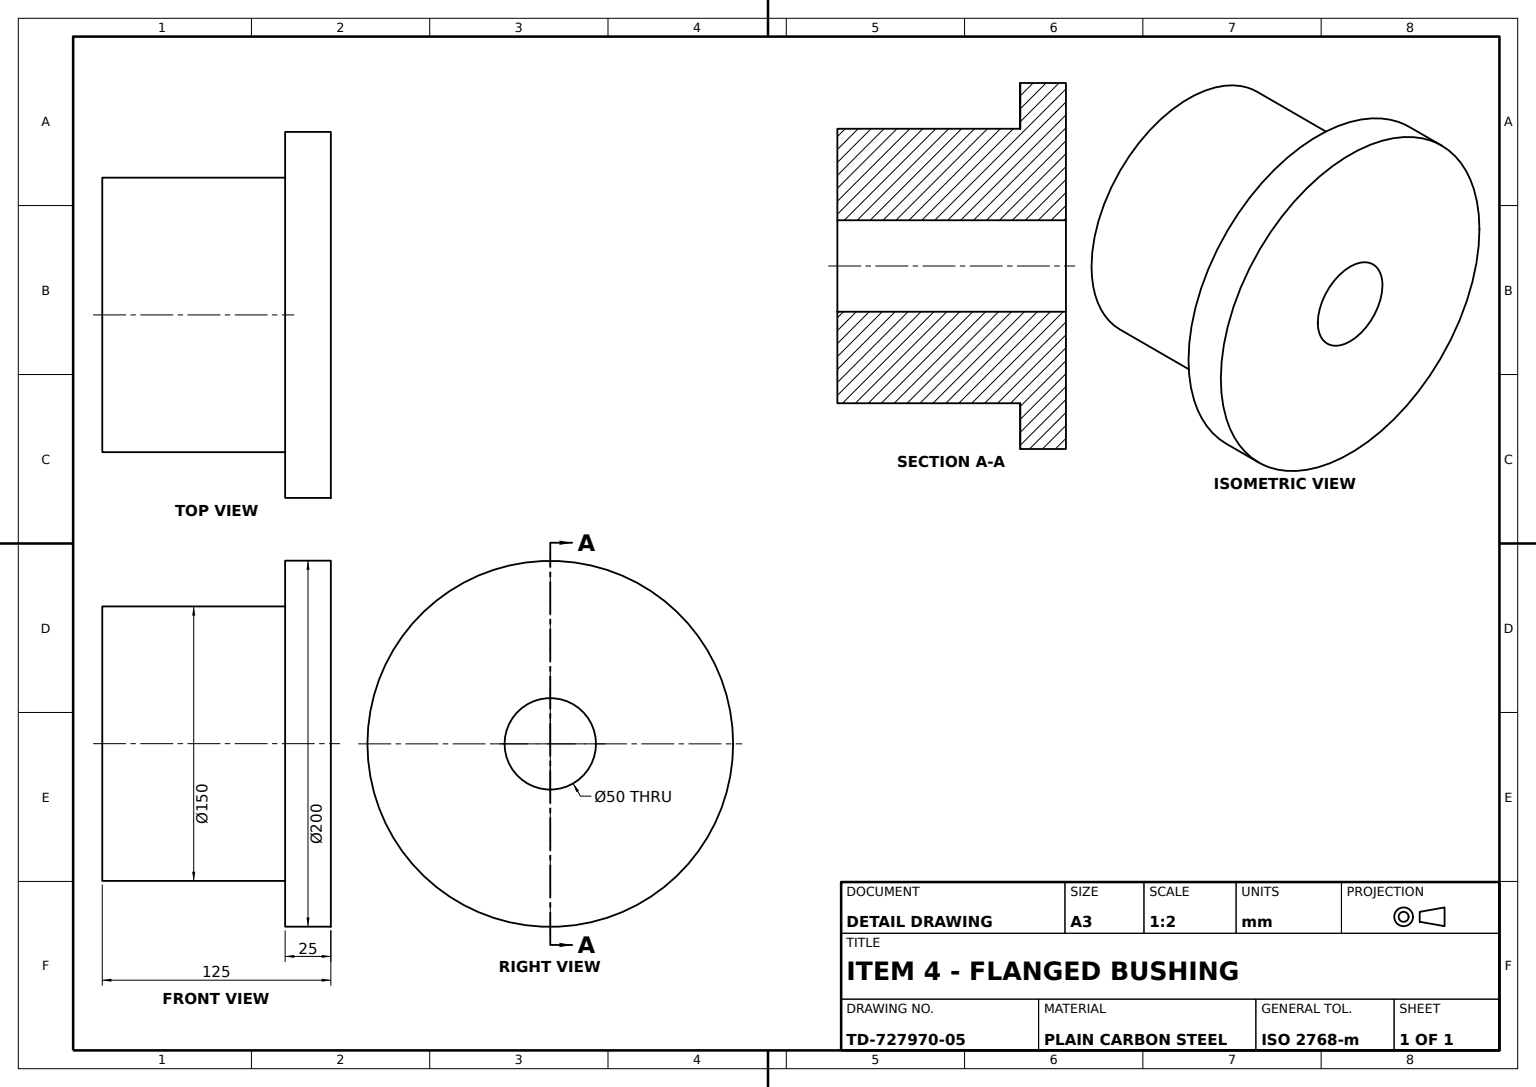
ISO-10303-21;
HEADER;
FILE_DESCRIPTION((''),'2;1');
FILE_NAME('','',(''),(''),'','','');
FILE_SCHEMA(('AUTOMOTIVE_DESIGN'));
ENDSEC;
DATA;
#1=APPLICATION_CONTEXT('');
#2=PRODUCT_CONTEXT('',#1,'mechanical');
#3=PRODUCT('','','',(#2));
#4=PRODUCT_DEFINITION_FORMATION('','',#3);
#5=PRODUCT_DEFINITION_CONTEXT('',#1,'design');
#6=PRODUCT_DEFINITION('','',#4,#5);
#7=PRODUCT_DEFINITION_SHAPE('','',#6);
#8=(LENGTH_UNIT()NAMED_UNIT(*)SI_UNIT(.MILLI.,.METRE.));
#9=(NAMED_UNIT(*)PLANE_ANGLE_UNIT()SI_UNIT($,.RADIAN.));
#10=(NAMED_UNIT(*)SI_UNIT($,.STERADIAN.)SOLID_ANGLE_UNIT());
#11=UNCERTAINTY_MEASURE_WITH_UNIT(LENGTH_MEASURE(1.E-05),#8,'distance_accuracy_value','');
#12=(GEOMETRIC_REPRESENTATION_CONTEXT(3)GLOBAL_UNCERTAINTY_ASSIGNED_CONTEXT((#11))GLOBAL_UNIT_ASSIGNED_CONTEXT((#8,#9,#10))REPRESENTATION_CONTEXT('',''));
#13=CARTESIAN_POINT('',(0.,100.,100.));
#14=VERTEX_POINT('',#13);
#15=CARTESIAN_POINT('',(0.,100.,-100.));
#16=VERTEX_POINT('',#15);
#17=CARTESIAN_POINT('',(0.,100.,0.));
#18=DIRECTION('',(0.,-1.,0.));
#19=DIRECTION('',(0.,0.,-1.));
#20=AXIS2_PLACEMENT_3D('',#17,#18,#19);
#21=CIRCLE('',#20,100.);
#22=EDGE_CURVE('',#14,#16,#21,.T.);
#23=ORIENTED_EDGE('',*,*,#22,.T.);
#24=EDGE_CURVE('',#16,#14,#21,.T.);
#25=ORIENTED_EDGE('',*,*,#24,.T.);
#26=EDGE_LOOP('',(#23,#25));
#27=FACE_OUTER_BOUND('',#26,.T.);
#28=CARTESIAN_POINT('',(0.,100.,75.));
#29=VERTEX_POINT('',#28);
#30=CARTESIAN_POINT('',(0.,100.,-75.));
#31=VERTEX_POINT('',#30);
#32=CIRCLE('',#20,75.);
#33=EDGE_CURVE('',#29,#31,#32,.T.);
#34=ORIENTED_EDGE('',*,*,#33,.F.);
#35=EDGE_CURVE('',#31,#29,#32,.T.);
#36=ORIENTED_EDGE('',*,*,#35,.F.);
#37=EDGE_LOOP('',(#34,#36));
#38=FACE_BOUND('',#37,.T.);
#39=CARTESIAN_POINT('',(100.,100.,0.));
#40=AXIS2_PLACEMENT_3D('',#39,#18,#19);
#41=PLANE('',#40);
#42=ADVANCED_FACE('',(#27,#38),#41,.T.);
#43=CARTESIAN_POINT('',(0.,0.,75.));
#44=VERTEX_POINT('',#43);
#45=CARTESIAN_POINT('',(0.,0.,-75.));
#46=VERTEX_POINT('',#45);
#47=CARTESIAN_POINT('',(0.,0.,0.));
#48=AXIS2_PLACEMENT_3D('',#47,#18,#19);
#49=CIRCLE('',#48,75.);
#50=EDGE_CURVE('',#44,#46,#49,.T.);
#51=ORIENTED_EDGE('',*,*,#50,.T.);
#52=EDGE_CURVE('',#46,#44,#49,.T.);
#53=ORIENTED_EDGE('',*,*,#52,.T.);
#54=EDGE_LOOP('',(#51,#53));
#55=FACE_OUTER_BOUND('',#54,.T.);
#56=CARTESIAN_POINT('',(0.,0.,25.));
#57=VERTEX_POINT('',#56);
#58=CARTESIAN_POINT('',(0.,0.,-25.));
#59=VERTEX_POINT('',#58);
#60=CIRCLE('',#48,25.);
#61=EDGE_CURVE('',#57,#59,#60,.T.);
#62=ORIENTED_EDGE('',*,*,#61,.F.);
#63=EDGE_CURVE('',#59,#57,#60,.T.);
#64=ORIENTED_EDGE('',*,*,#63,.F.);
#65=EDGE_LOOP('',(#62,#64));
#66=FACE_BOUND('',#65,.T.);
#67=CARTESIAN_POINT('',(75.,0.,0.));
#68=AXIS2_PLACEMENT_3D('',#67,#18,#19);
#69=PLANE('',#68);
#70=ADVANCED_FACE('',(#55,#66),#69,.T.);
#71=CARTESIAN_POINT('',(0.,125.,100.));
#72=VERTEX_POINT('',#71);
#73=CARTESIAN_POINT('',(0.,0.,100.));
#74=VECTOR('',#18,1000.);
#75=LINE('',#73,#74);
#76=EDGE_CURVE('',#72,#14,#75,.T.);
#77=ORIENTED_EDGE('',*,*,#76,.T.);
#78=ORIENTED_EDGE('',*,*,#24,.F.);
#79=CARTESIAN_POINT('',(0.,125.,-100.));
#80=VERTEX_POINT('',#79);
#81=CARTESIAN_POINT('',(0.,0.,-100.));
#82=LINE('',#81,#74);
#83=EDGE_CURVE('',#80,#16,#82,.T.);
#84=ORIENTED_EDGE('',*,*,#83,.F.);
#85=CARTESIAN_POINT('',(0.,125.,0.));
#86=AXIS2_PLACEMENT_3D('',#85,#18,#19);
#87=CIRCLE('',#86,100.);
#88=EDGE_CURVE('',#80,#72,#87,.T.);
#89=ORIENTED_EDGE('',*,*,#88,.T.);
#90=EDGE_LOOP('',(#77,#78,#84,#89));
#91=FACE_OUTER_BOUND('',#90,.T.);
#92=CYLINDRICAL_SURFACE('',#48,100.);
#93=ADVANCED_FACE('',(#91),#92,.T.);
#94=CARTESIAN_POINT('',(0.,125.,-25.));
#95=VERTEX_POINT('',#94);
#96=CARTESIAN_POINT('',(0.,125.,25.));
#97=VERTEX_POINT('',#96);
#98=CIRCLE('',#86,25.);
#99=EDGE_CURVE('',#95,#97,#98,.T.);
#100=ORIENTED_EDGE('',*,*,#99,.F.);
#101=LINE('',#58,#74);
#102=EDGE_CURVE('',#95,#59,#101,.T.);
#103=ORIENTED_EDGE('',*,*,#102,.T.);
#104=ORIENTED_EDGE('',*,*,#63,.T.);
#105=LINE('',#56,#74);
#106=EDGE_CURVE('',#97,#57,#105,.T.);
#107=ORIENTED_EDGE('',*,*,#106,.F.);
#108=EDGE_LOOP('',(#100,#103,#104,#107));
#109=FACE_OUTER_BOUND('',#108,.T.);
#110=CYLINDRICAL_SURFACE('',#48,25.);
#111=ADVANCED_FACE('',(#109),#110,.F.);
#112=LINE('',#45,#74);
#113=EDGE_CURVE('',#31,#46,#112,.T.);
#114=ORIENTED_EDGE('',*,*,#113,.F.);
#115=ORIENTED_EDGE('',*,*,#35,.T.);
#116=LINE('',#43,#74);
#117=EDGE_CURVE('',#29,#44,#116,.T.);
#118=ORIENTED_EDGE('',*,*,#117,.T.);
#119=ORIENTED_EDGE('',*,*,#52,.F.);
#120=EDGE_LOOP('',(#114,#115,#118,#119));
#121=FACE_OUTER_BOUND('',#120,.T.);
#122=CYLINDRICAL_SURFACE('',#48,75.);
#123=ADVANCED_FACE('',(#121),#122,.T.);
#124=ORIENTED_EDGE('',*,*,#102,.F.);
#125=EDGE_CURVE('',#97,#95,#98,.T.);
#126=ORIENTED_EDGE('',*,*,#125,.F.);
#127=ORIENTED_EDGE('',*,*,#106,.T.);
#128=ORIENTED_EDGE('',*,*,#61,.T.);
#129=EDGE_LOOP('',(#124,#126,#127,#128));
#130=FACE_OUTER_BOUND('',#129,.T.);
#131=ADVANCED_FACE('',(#130),#110,.F.);
#132=ORIENTED_EDGE('',*,*,#33,.T.);
#133=ORIENTED_EDGE('',*,*,#113,.T.);
#134=ORIENTED_EDGE('',*,*,#50,.F.);
#135=ORIENTED_EDGE('',*,*,#117,.F.);
#136=EDGE_LOOP('',(#132,#133,#134,#135));
#137=FACE_OUTER_BOUND('',#136,.T.);
#138=ADVANCED_FACE('',(#137),#122,.T.);
#139=ORIENTED_EDGE('',*,*,#88,.F.);
#140=EDGE_CURVE('',#72,#80,#87,.T.);
#141=ORIENTED_EDGE('',*,*,#140,.F.);
#142=EDGE_LOOP('',(#139,#141));
#143=FACE_OUTER_BOUND('',#142,.T.);
#144=ORIENTED_EDGE('',*,*,#125,.T.);
#145=ORIENTED_EDGE('',*,*,#99,.T.);
#146=EDGE_LOOP('',(#144,#145));
#147=FACE_BOUND('',#146,.T.);
#148=CARTESIAN_POINT('',(25.,125.,0.));
#149=DIRECTION('',(0.,1.,0.));
#150=DIRECTION('',(0.,0.,1.));
#151=AXIS2_PLACEMENT_3D('',#148,#149,#150);
#152=PLANE('',#151);
#153=ADVANCED_FACE('',(#143,#147),#152,.T.);
#154=ORIENTED_EDGE('',*,*,#22,.F.);
#155=ORIENTED_EDGE('',*,*,#76,.F.);
#156=ORIENTED_EDGE('',*,*,#140,.T.);
#157=ORIENTED_EDGE('',*,*,#83,.T.);
#158=EDGE_LOOP('',(#154,#155,#156,#157));
#159=FACE_OUTER_BOUND('',#158,.T.);
#160=ADVANCED_FACE('',(#159),#92,.T.);
#161=CLOSED_SHELL('',(#42,#70,#93,#111,#123,#131,#138,#153,#160));
#162=MANIFOLD_SOLID_BREP('',#161);
#163=ADVANCED_BREP_SHAPE_REPRESENTATION('',(#162),#12);
#164=SHAPE_DEFINITION_REPRESENTATION(#7,#163);
ENDSEC;
END-ISO-10303-21;
